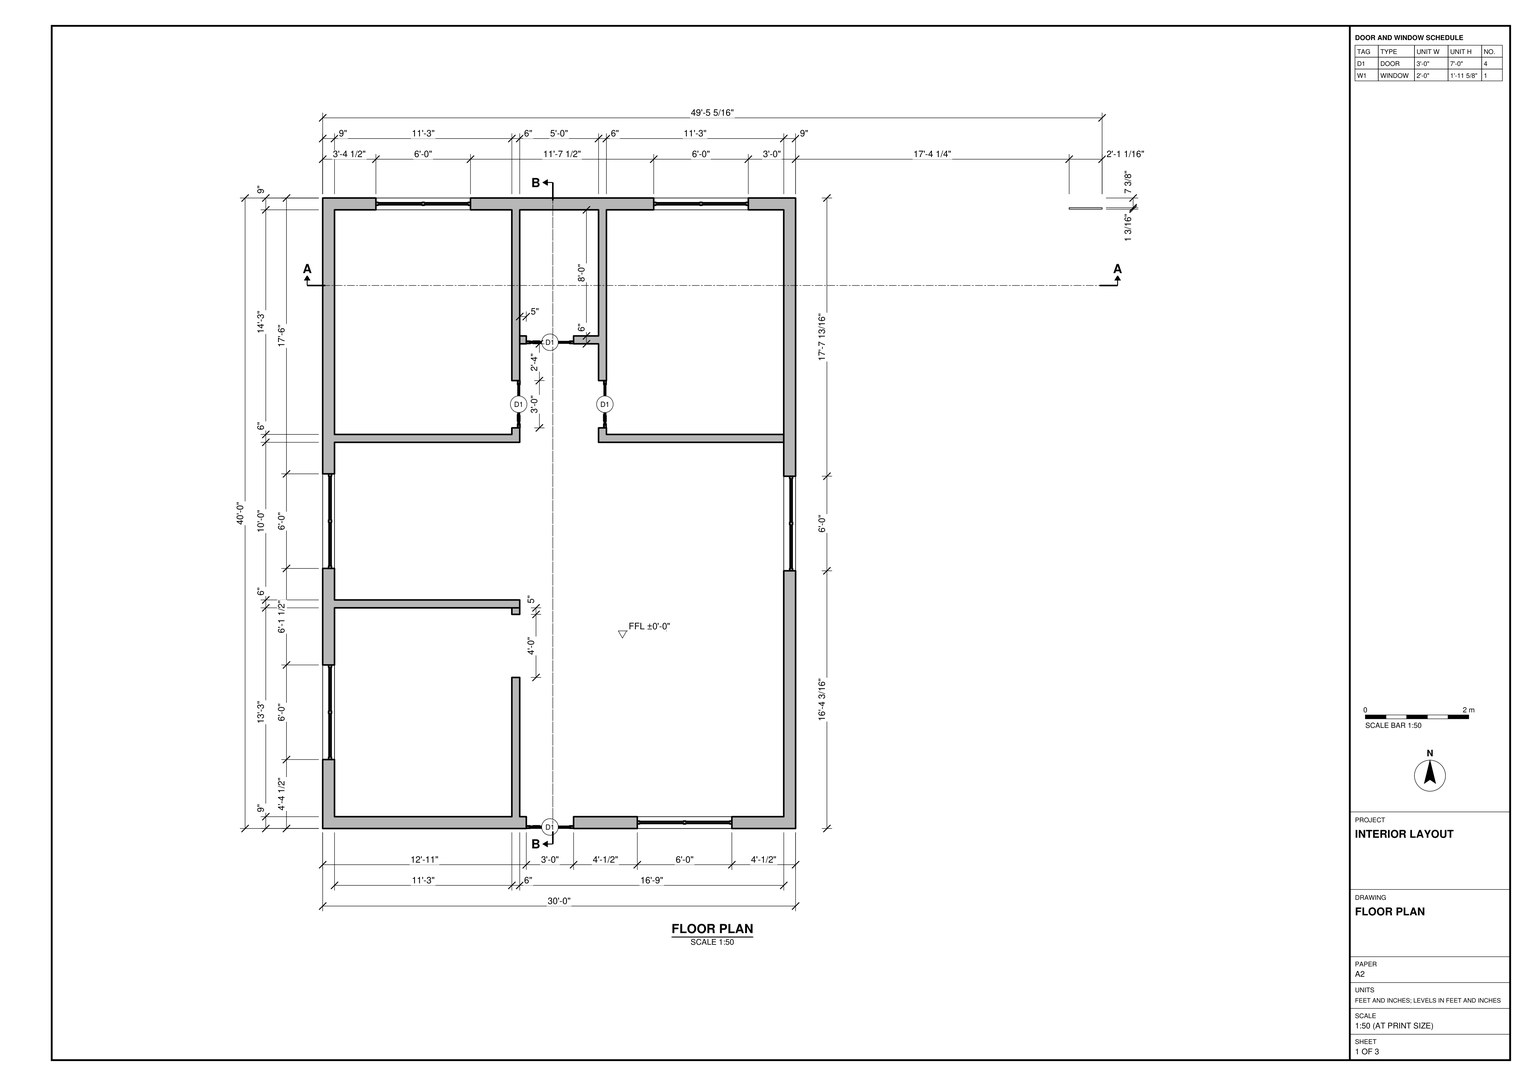
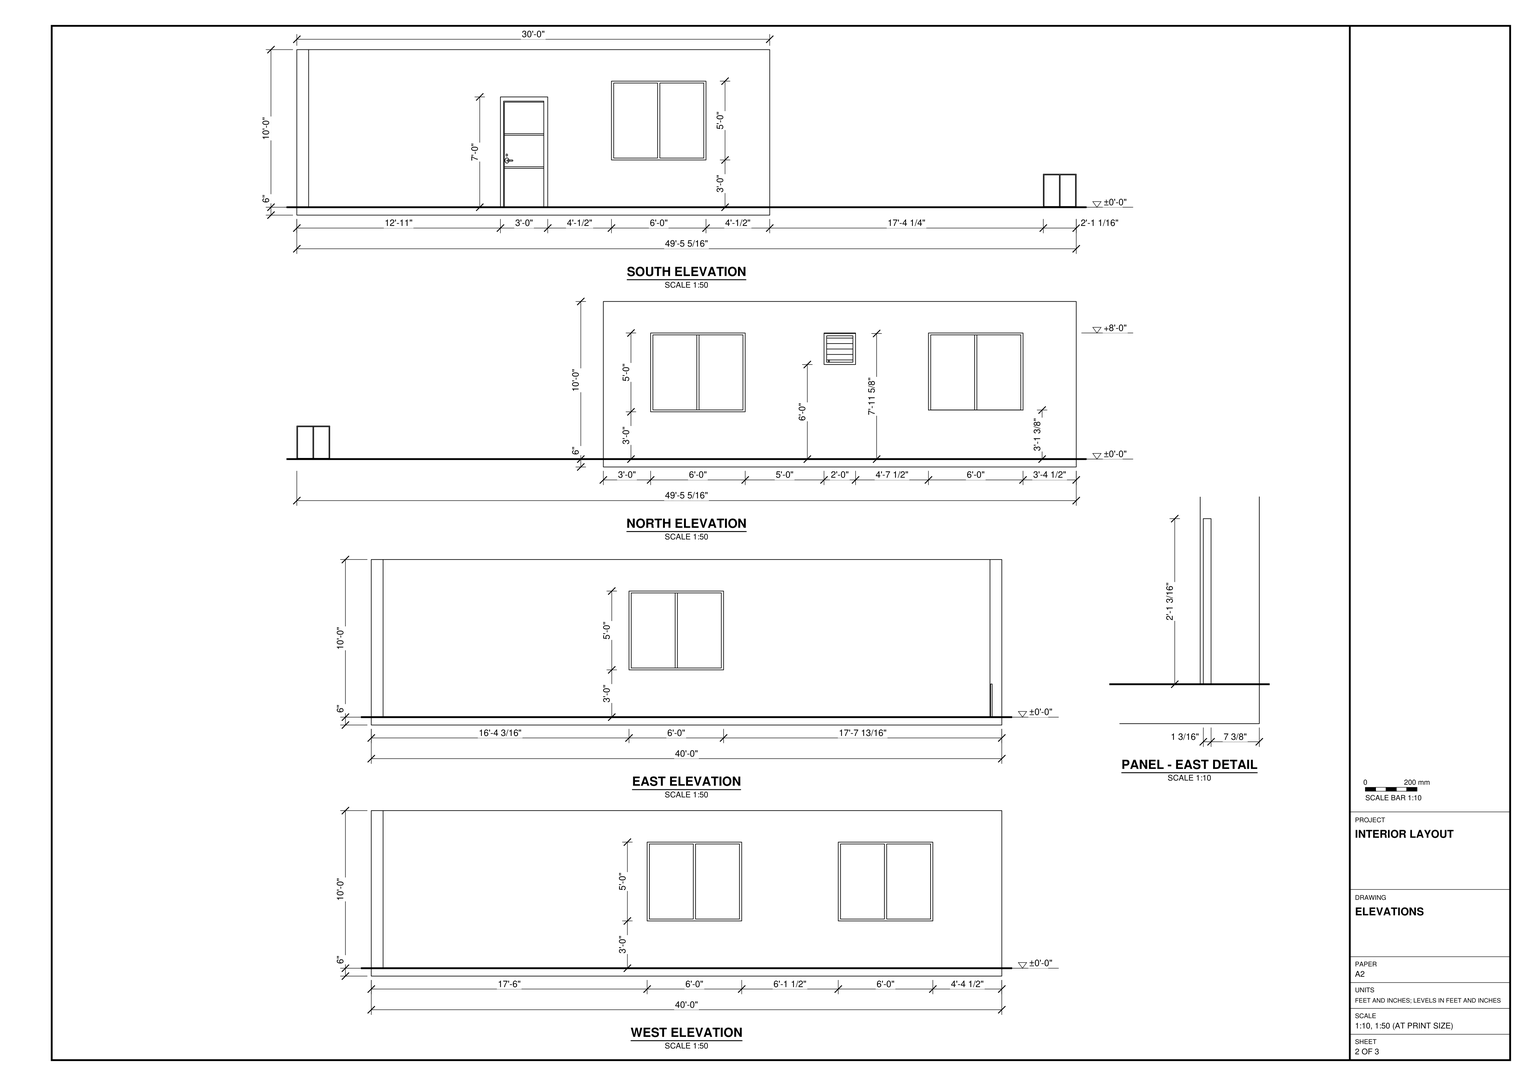
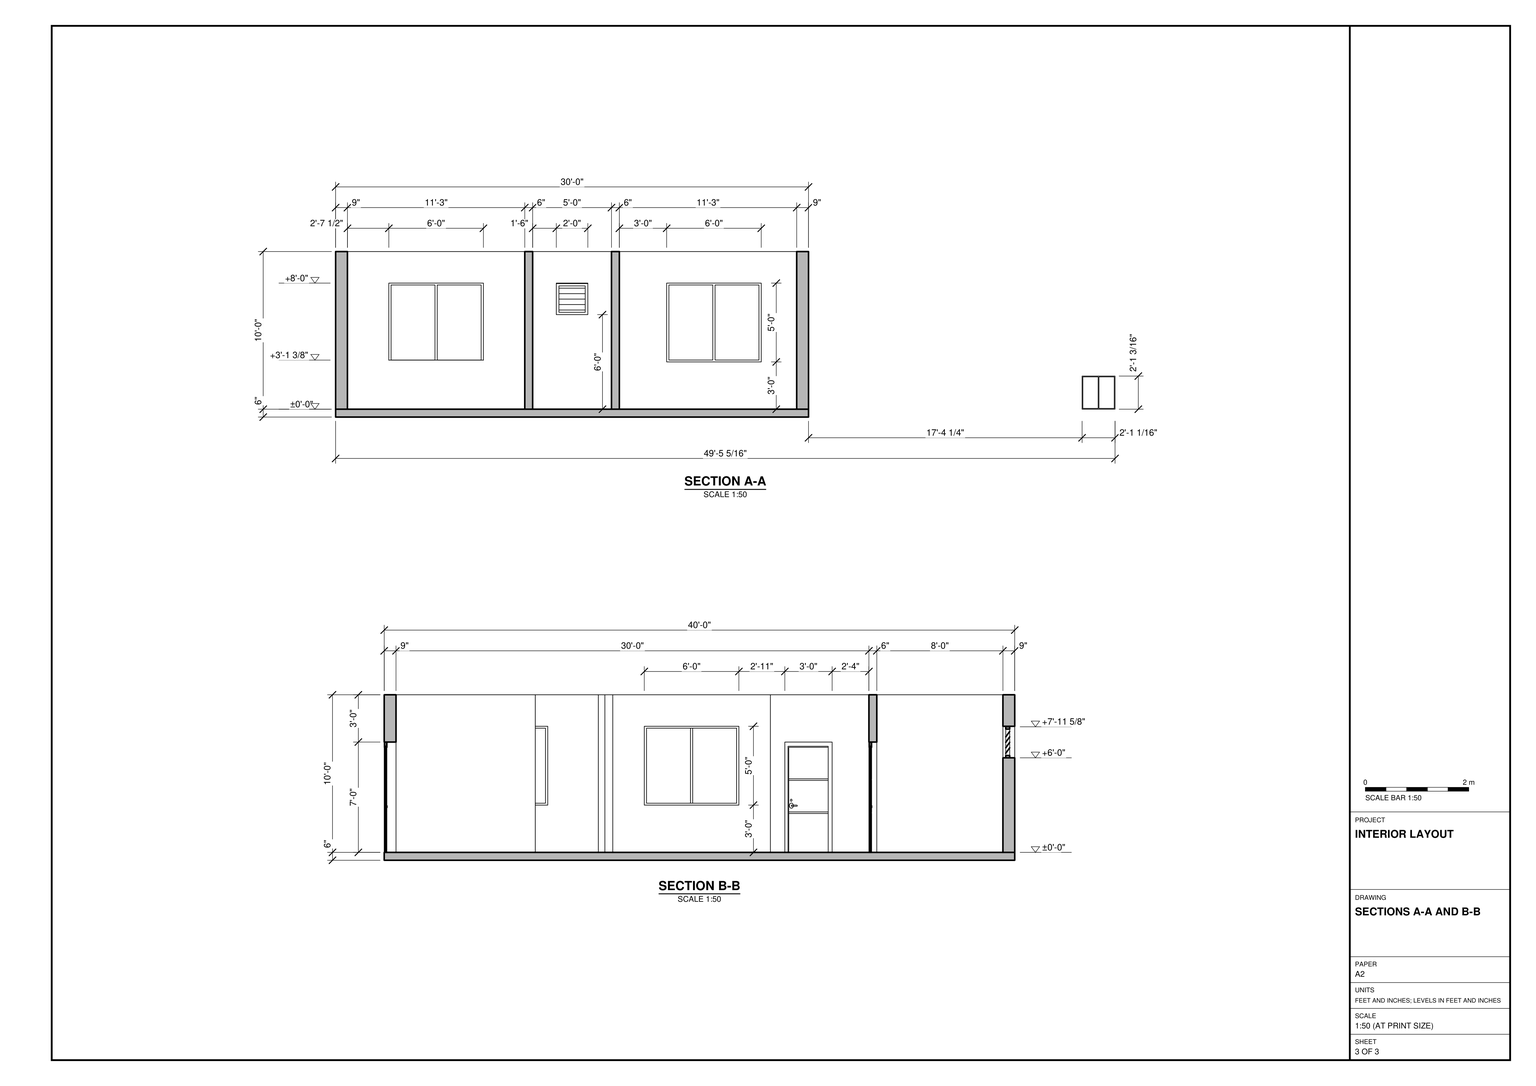
Work in feet and inches in SketchUp. Use task_files/diagram_01.pdf to model the floor plan, using the elevations and sections to set wall, door, window and panel heights. The main shell has a rectangular footprint of 30'-0" by 40'-0". Including the detached panel to the east, the overall model measures 49'-5 5/16" east to west, 40'-0" north to south and 10'-6" high.

Set the finished floor at ±0'-0", with the 6" slab below it. Raise the walls 10'-0" above the floor, using 9" exterior walls and 6" interior partitions. At the north end, form two rooms flanking a narrower central room. Place their three doors off the common passage. Follow the partition returns around the southwest room, leaving its access open to the larger space on the east. Leave the shell open at the top as shown in section.

Place the entrance in the south wall with a wide window to its east. Use the elevations to position the other wide windows and the small high ventilating window. Set the detached upright panel near the north end of the east wall, using the plan for its offset and the east detail for its profile.

Keep shell elements and the detached panel in separate groups or components, and use components for repeated parts. Any decor or loose items may use suitable library components. Save one SketchUp model as output_files/single_storey_interior_layout_and_detached_east_panel.skp.

# SketchUp Ruby script. Lengths in inches.
U = 1.inch
M = Sketchup.active_model
def pt(a) = Geom::Point3d.new(a.map { |v| v * U })
def face(e, loops, mat)
  f = e.add_face(loops[0].map { |a| pt(a) })
  loops[1..].each { |l| e.add_face(l.map { |a| pt(a) }).erase! }
  f.material = f.back_material = mat if mat
  f
end
# faces: each face lists its corners as indices into pts; further lists are holes
def faces(e, pts, list, mat = nil) = list.each { |f| face(e, (f[0].is_a?(Array) ? f : [f]).map { |l| l.map { |i| pts[i] } }, mat) }
# xy, xz, yz: faces in a plane at the given z, y or x. An outline is a flat list of corners, or four numbers for a rectangle; further outlines are holes
def ring(l) = l.size == 4 ? [[l[0], l[1]], [l[2], l[1]], [l[2], l[3]], [l[0], l[3]]] : l.each_slice(2).to_a
def flat(e, list, mat, &to3) = list.each { |f| face(e, (f[0].is_a?(Array) ? f : [f]).map { |l| ring(l).map { |u, v| to3.(u, v) } }, mat) }
def xy(e, z, list, mat = nil) = flat(e, list, mat) { |x, y| [x, y, z] }
def xz(e, y, list, mat = nil) = flat(e, list, mat) { |x, z| [x, y, z] }
def yz(e, x, list, mat = nil) = flat(e, list, mat) { |y, z| [x, y, z] }
def lines(e, pts, list) = list.each { |a, b| e.add_line(pt(pts[a]), pt(pts[b])) }
# prism: a flat outline (further loops are holes) pulled along v
def prism(e, loops, v, mat = nil)
  f = face(e, loops, mat); d = Geom::Vector3d.new(v.map { |x| x * U })
  f.pushpull(f.normal.samedirection?(d) ? d.length : -d.length)
end
def box(e, o, s, mat = nil) = prism(e, [[o, [o[0] + s[0], o[1], o[2]], [o[0] + s[0], o[1] + s[1], o[2]], [o[0], o[1] + s[1], o[2]]]], [0, 0, s[2]], mat)
def at(x, y, z, deg = 0) = Geom::Transformation.translation(pt([x, y, z])) * Geom::Transformation.rotation(ORIGIN, Z_AXIS, deg.degrees)
def axes(o, x, y, z) = Geom::Transformation.new([*x, 0, *y, 0, *z, 0, *pt(o).to_a, 1])
def part(name) = M.definitions.add(name)
# library, detail: a bought-in or finely detailed component or shape, given as its bounding box
def library(name, o, s) = part(name).tap { |d| box(d.entities, o, s) }
def detail(e, o, s) = box(e.add_group.entities, o, s)
def put(e, d, t, mat = nil) = e.add_instance(d, t).tap { |i| i.material = mat if mat }
def group(e, t, mat = nil) = e.add_group.tap { |g| g.transformation = t; g.material = mat if mat }.entities
root = M.entities
M.materials.add("[Color_008]").color = [30, 30, 30]
M.materials.add("[Color_009]").color = [0, 0, 0]
M.materials.add("[Translucent Glass Gray]").color = [128, 128, 128]
M.materials["[Translucent Glass Gray]"].alpha = 0.5
M.materials.add("[Translucent Glass Tinted]1").color = [7, 201, 240]
M.materials["[Translucent Glass Tinted]1"].alpha = 0.48
M.materials.add("[Translucent_Glass_Gray]").color = [128, 128, 128]
M.materials["[Translucent_Glass_Gray]"].alpha = 0.5
M.materials.add("[Wood Cherry Original]").color = [152, 86, 42]
M.materials.add("[Wood Floor Parquet]").color = [145, 89, 39]
c1 = part("Group\#2")
xy(c1.entities,0,[[0,0,82.68,1.18]],"[Color_009]")
xy(c1.entities,1.97,[[1.97,0.98,40.35,1.18],[42.32,0.98,80.71,1.18]])
xy(c1.entities,1.97,[[1.97,0,40.35,0.3],[42.32,0,80.71,0.3]],"[Color_009]")
xy(c1.entities,80.71,[[1.97,0,40.35,0.3],[42.32,0,80.71,0.3],[1.97,0.3,40.35,0.98],[42.32,0.3,80.71,0.98],[1.97,0.98,40.35,1.18],
  [42.32,0.98,80.71,1.18]])
xy(c1.entities,82.68,[[0,0,82.68,1.18]],"[Color_008]")
xz(c1.entities,0,[[[0,0,82.68,82.68],[1.97,1.97,40.35,80.71],[42.32,1.97,80.71,80.71]]],"[Color_009]")
xz(c1.entities,0.3,[[1.97,1.97,40.35,80.71],[42.32,1.97,80.71,80.71]],"[Translucent_Glass_Gray]")
xz(c1.entities,0.98,[[1.97,1.97,40.35,80.71],[42.32,1.97,80.71,80.71]],"[Translucent_Glass_Gray]")
xz(c1.entities,1.18,[[[0,0,82.68,82.68],[1.97,1.97,80.71,80.71]],[40.35,1.97,42.32,80.71]],"[Color_009]")
yz(c1.entities,0,[[0,0,1.18,82.68]],"[Color_009]")
yz(c1.entities,1.97,[[0.98,1.97,1.18,80.71]])
yz(c1.entities,1.97,[[0,1.97,0.3,80.71]],"[Color_009]")
yz(c1.entities,40.35,[[0,1.97,0.3,80.71],[0.98,1.97,1.18,80.71]],"[Color_009]")
yz(c1.entities,42.32,[[0,1.97,0.3,80.71],[0.98,1.97,1.18,80.71]])
yz(c1.entities,80.71,[[0,1.97,0.3,80.71],[0.98,1.97,1.18,80.71]],"[Color_009]")
yz(c1.entities,82.68,[[0,0,1.18,82.68]],"[Color_009]")
c2 = library("main+door",[0,-0.79,0],[47.24,7.88,82.68])
c3 = part("ventilator")
g1 = group(c3.entities,at(0,0,0))
xy(g1,0,[[0,0,24,1],[0,1,24,6.83]],"[Wood Floor Parquet]")
xy(g1,1.75,[[2,0,22,6.83]],"[Wood Floor Parquet]")
xy(g1,21.87,[[2,0,22,6.83]],"[Wood Cherry Original]")
xy(g1,23.62,[[0,0,24,1],[0,1,24,6.83]],"[Wood Floor Parquet]")
xz(g1,0,[[[0,0,24,23.62],[2,1.75,22,21.87]]],"[Wood Floor Parquet]")
xz(g1,6.83,[[[0,0,24,23.62],[2,1.75,22,21.87]]],"[Wood Cherry Original]")
yz(g1,0,[[0,0,1,23.62],[1,0,6.83,23.62]],"[Wood Floor Parquet]")
yz(g1,2,[[0,1.75,6.83,1.75,6.83,7.66,0,3.5],[0,3.5,6.83,7.66,6.83,11.8125,0,7.66],[0,7.66,6.83,11.8125,6.83,15.97,0,11.8125],[0,11.8125,6.83,15.97,6.83,20.12,0,15.97],[0,15.97,6.83,20.12,6.83,21.87,0,21.87]],"[Wood Floor Parquet]")
yz(g1,22,[[0,1.75,0,3.5,6.83,7.66,6.83,1.75],[0,3.5,0,7.66,6.83,11.8125,6.83,7.66],[0,7.66,0,11.8125,6.83,15.97,6.83,11.8125],[0,11.8125,0,15.97,6.83,20.12,6.83,15.97],[0,15.97,0,21.87,6.83,21.87,6.83,20.12]],"[Wood Floor Parquet]")
yz(g1,24,[[0,0,1,23.62],[1,0,6.83,23.62]],"[Wood Floor Parquet]")
p = [[2,0,3.5],[2,6.83,7.66],[22,6.83,7.66],[22,0,3.5],[2,6.83,11.8125],[2,0,7.66],
  [22,0,7.66],[22,6.83,11.8125],[2,0,11.8125],[2,6.83,15.97],[22,6.83,15.97],[22,0,11.8125],
  [2,6.83,20.12],[2,0,15.97],[22,0,15.97],[22,6.83,20.12]]
faces(g1,p,[[0,1,2,3],[4,5,6,7],[8,9,10,11]],"[Translucent Glass Tinted]1")
faces(g1,p,[[12,13,14,15]],"[Translucent Glass Gray]")
c4 = library("Group\#1",[0,0,0],[360,480,0.01])
p = [[114.06,161,0],[114,161,0],[490.97,448.77,60.44],[490.97,448.69,60.37],[490.96,448.59,60.16],[490.96,448.59,60.09],
  [490.96,448.62,60.25],[490.96,448.62,59.97],[490.97,448.74,59.92],[491.07,449.91,60.75],[491.08,450,60.51],[491.08,450.01,60.11],
  [491.08,449.94,60.01],[491.02,449.31,61.79],[491.05,449.59,61.33],[491.0625,449.78,59.97],[491.08,450.04,60.33],[491.0625,449.78,60.9375]]
lines(root,p,[[0,1],[2,3],[4,5],[3,6],[7,8],[5,7],[6,4],[9,10],[11,12],[13,14],[12,15],[11,16],
  [17,9],[17,14],[16,10]])
put(root,c1,axes([568.25,471.47,0],[0.3034,0,0],[0,1,0],[0,0,0.305]))
put(root,c1,axes([4.5,124.5,36],[0,-0.87086,0],[1.85,0,0],[0,0,0.72571]))
g2 = group(root,at(0,0,0))
xy(g2,0,[[191,0,311.5,9],[311.5,0,360,9],[351,9,360,268.19],[0,52.5,9,124.5],[0,124.5,9,270],
  [144,163,150,168],[9,168,150,174],[351,268.19,360,471],[210,294,351,300],[210,300,216,305],
  [144,341,150,480],[150,369,155,375],[0,471,112.5,480],[112.5,471,144,480],[150,471,192,480],
  [192,471,210,480],[252,471,324,480]])
xy(g2,36,[[239.5,0,311.5,9],[0,52.5,9,124.5],[351,196.19,360,268.19],[0,198,9,270],[252,471,324,480]])
xy(g2,37.36,[[40.5,471,112.5,480]])
xy(g2,72,[[168,471,192,480]])
xy(g2,84,[[155,0,191,9],[144,305,150,341],[210,305,216,341],[155,369,191,375]])
xy(g2,96,[[239.5,0,311.5,9],[0,52.5,9,124.5],[351,196.19,360,268.19],[0,198,9,270],[40.5,471,112.5,480],
  [168,471,192,480],[252,471,324,480]])
xy(g2,120,[[0,0,360,0,360,471,351,471,351,9,9,9,9,168,150,168,150,174,9,174,9,294,150,294,150,471,210,471,210,375,150,375,150,369,210,369,210,294,351,294,351,300,216,300,216,471,360,471,360,480,0,480,0,471,144,471,144,300,9,300,9,471,0,471],[144,9,150,115],[144,163,150,168]])
xz(g2,0,[[0,0,9,120],[[9,0,155,0,155,84,191,84,191,0,360,0,360,120,9,120],[239.5,36,311.5,96]]])
xz(g2,9,[[9,0,144,120],[[150,0,150,120,351,120,351,0,191,0,191,84,155,84,155,0],[239.5,36,311.5,96]]])
xz(g2,52.5,[[0,36,9,96]])
xz(g2,115,[[144,0,150,120]])
xz(g2,124.5,[[0,36,9,96]])
xz(g2,163,[[144,0,150,120]])
xz(g2,168,[[9,0,144,120],[144,0,150,120]])
xz(g2,174,[[9,0,150,120]])
xz(g2,196.19,[[351,36,360,96]])
xz(g2,198,[[0,36,9,96]])
xz(g2,268.19,[[351,36,360,96]])
xz(g2,270,[[0,36,9,96]])
xz(g2,294,[[9,0,144,120],[144,0,150,120],[210,0,351,120]])
xz(g2,300,[[9,0,144,120],[216,0,351,120]])
xz(g2,305,[[144,0,150,84],[210,0,216,84]])
xz(g2,341,[[144,0,150,84],[210,0,216,84]])
xz(g2,369,[[150,0,155,0,155,84,191,84,191,0,210,0,210,120,150,120]])
xz(g2,375,[[150,0,150,120,210,120,210,0,191,0,191,84,155,84,155,0]])
xz(g2,471,[[[9,0,144,120],[40.5,37.36,112.5,96]],[[150,0,210,120],[168,72,192,96]],[[216,0,351,120],[252,36,324,96]]])
xz(g2,480,[[[0,0,360,120],[252,36,324,96],[40.5,37.36,112.5,96],[168,72,192,96]]])
yz(g2,0,[[[0,0,471,120],[198,36,270,96],[52.5,36,124.5,96]],[471,0,480,120]])
yz(g2,9,[[[9,0,168,120],[52.5,36,124.5,96]],[[174,0,294,120],[198,36,270,96]],[300,0,471,120]])
yz(g2,40.5,[[471,37.36,480,96]])
yz(g2,112.5,[[471,37.36,480,96]])
yz(g2,144,[[9,0,115,120],[163,0,168,120],[300,0,300,120,471,120,471,0,341,0,341,84,305,84,305,0]])
yz(g2,150,[[9,0,115,120],[163,0,168,120],[168,0,174,120],[294,0,305,0,305,84,341,84,341,0,369,0,369,120,294,120],[369,0,375,120],
  [375,0,471,120]])
yz(g2,155,[[0,0,9,84],[369,0,375,84]])
yz(g2,168,[[471,72,480,96]])
yz(g2,191,[[0,0,9,84],[369,0,375,84]])
yz(g2,192,[[471,72,480,96]])
yz(g2,210,[[294,0,294,120,369,120,369,0,341,0,341,84,305,84,305,0],[375,0,471,120]])
yz(g2,216,[[300,0,305,0,305,84,341,84,341,0,471,0,471,120,300,120]])
yz(g2,239.5,[[0,36,9,96]])
yz(g2,252,[[471,36,480,96]])
yz(g2,311.5,[[0,36,9,96]])
yz(g2,324,[[471,36,480,96]])
yz(g2,351,[[[9,0,294,120],[196.19,36,268.19,96]],[294,0,300,120],[300,0,471,120]])
yz(g2,360,[[0,0,9,120],[[9,0,471,120],[196.19,36,268.19,96]],[471,0,480,120]])
put(g2,c2,axes([150.14,305,0],[0,0.762,0],[-0.3,0,0],[0,0,1.016]))
put(g2,c2,axes([215.76,305,0],[0,0.762,0],[-0.3,0,0],[0,0,1.016]))
put(g2,c3,axes([168,473.17,72],[1,0,0],[0,0.44,0],[0,0,1]))
put(g2,c2,axes([155,369.24,0],[0.762,0,0],[0,0.3,0],[0,0,1.016]))
put(g2,c2,axes([155,0.24,0],[0.762,0,0],[0,0.3,0],[0,0,1.016]))
put(g2,c1,axes([4.5,270,36],[0,-0.87086,0],[1.85,0,0],[0,0,0.72571]))
put(g2,c1,axes([252,474.5,36],[0.87086,0,0],[0,1.85,0],[0,0,0.72571]))
put(g2,c1,axes([355.5,268.19,36],[0,-0.87086,0],[1.85,0,0],[0,0,0.72571]))
put(g2,c1,axes([239.5,3.5,36],[0.87086,0,0],[0,1.85,0],[0,0,0.72571]))
put(g2,c1,axes([40.5,474.5,36],[0.87086,0,0],[0,1.85,0],[0,0,0.72571]))
g3 = group(root,at(0,0,-6))
box(g3,[0,0,0],[360,480,6])
put(root,c4,at(0,0,0))
